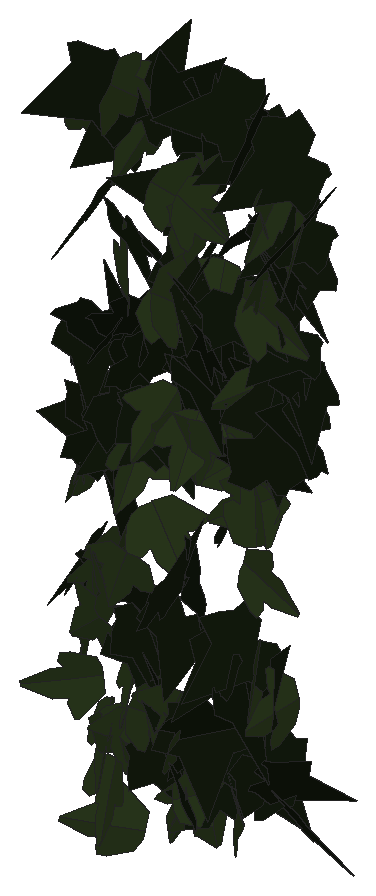
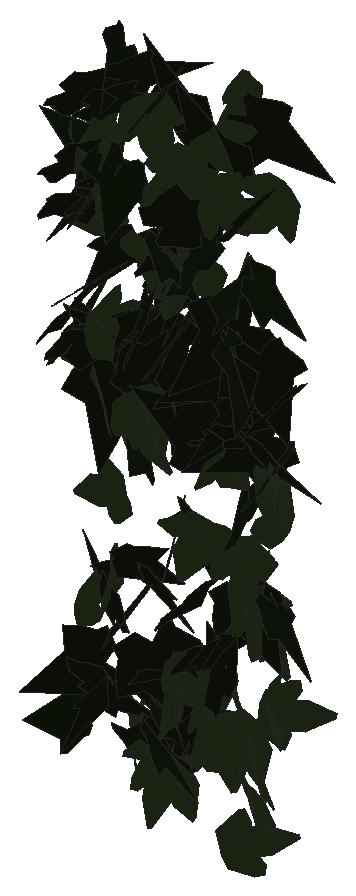
# SketchUp Ruby script. Lengths in inches.
U = 1.inch
M = Sketchup.active_model
def pt(a) = Geom::Point3d.new(a.map { |v| v * U })
def face(e, loops, mat)
  f = e.add_face(loops[0].map { |a| pt(a) })
  loops[1..].each { |l| e.add_face(l.map { |a| pt(a) }).erase! }
  f.material = f.back_material = mat if mat
  f
end
# faces: each face lists its corners as indices into pts; further lists are holes
def faces(e, pts, list, mat = nil) = list.each { |f| face(e, (f[0].is_a?(Array) ? f : [f]).map { |l| l.map { |i| pts[i] } }, mat) }
# xy, xz, yz: faces in a plane at the given z, y or x. An outline is a flat list of corners, or four numbers for a rectangle; further outlines are holes
def ring(l) = l.size == 4 ? [[l[0], l[1]], [l[2], l[1]], [l[2], l[3]], [l[0], l[3]]] : l.each_slice(2).to_a
def flat(e, list, mat, &to3) = list.each { |f| face(e, (f[0].is_a?(Array) ? f : [f]).map { |l| ring(l).map { |u, v| to3.(u, v) } }, mat) }
def xy(e, z, list, mat = nil) = flat(e, list, mat) { |x, y| [x, y, z] }
def xz(e, y, list, mat = nil) = flat(e, list, mat) { |x, z| [x, y, z] }
def yz(e, x, list, mat = nil) = flat(e, list, mat) { |y, z| [x, y, z] }
def lines(e, pts, list) = list.each { |a, b| e.add_line(pt(pts[a]), pt(pts[b])) }
# prism: a flat outline (further loops are holes) pulled along v
def prism(e, loops, v, mat = nil)
  f = face(e, loops, mat); d = Geom::Vector3d.new(v.map { |x| x * U })
  f.pushpull(f.normal.samedirection?(d) ? d.length : -d.length)
end
def box(e, o, s, mat = nil) = prism(e, [[o, [o[0] + s[0], o[1], o[2]], [o[0] + s[0], o[1] + s[1], o[2]], [o[0], o[1] + s[1], o[2]]]], [0, 0, s[2]], mat)
def at(x, y, z, deg = 0) = Geom::Transformation.translation(pt([x, y, z])) * Geom::Transformation.rotation(ORIGIN, Z_AXIS, deg.degrees)
def axes(o, x, y, z) = Geom::Transformation.new([*x, 0, *y, 0, *z, 0, *pt(o).to_a, 1])
def part(name) = M.definitions.add(name)
# library, detail: a bought-in or finely detailed component or shape, given as its bounding box
def library(name, o, s) = part(name).tap { |d| box(d.entities, o, s) }
def detail(e, o, s) = box(e.add_group.entities, o, s)
def put(e, d, t, mat = nil) = e.add_instance(d, t).tap { |i| i.material = mat if mat }
def group(e, t, mat = nil) = e.add_group.tap { |g| g.transformation = t; g.material = mat if mat }.entities
root = M.entities
M.materials.add("efeu1").color = [18, 25, 13]
M.materials.add("efeu2").color = [43, 57, 29]
c1 = part("ivyleaf_9")
p = [[1.54,2.16,1.25],[1.36,2.04,1.19],[-0.21,0.99,0.68],[-0.71,1.11,0.82],[-0.85,0.86,0.67],[-0.8,0.17,0.21],
  [-0.9,-0.01,0.1],[-0.67,-0.16,-0.02],[-0.08,-0.08,-0.05],[-0.03,-0.6,-0.4],[0.65,-0.88,-0.66],[0.83,-0.6,-0.49],
  [1.29,-0.42,-0.43],[1.8125,-0.07,-0.26],[1.21,0.44,0.15]]
faces(c1.entities,p,[[0,1,2,3,4,5,6,7,8,9,10,11,12,13,14]],"efeu1")
c2 = part("ivyleaf_10")
p = [[0,0.5,-0.03],[-0.0625,2.02,-0.43],[-0.19,2.01,-0.46],[-0.54,1.05,-0.29],[-0.52,0.625,-0.18],[-0.83,0.76,-0.28],
  [-1.16,0.64,-0.33],[-1.15,0.33,-0.24],[-0.77,-0.39,0.02],[-0.3,-0.51,0.16],[0.04,-0.48,0.23],[-0.02,2.01,-0.4375],
  [-0.06,2.01,-0.43],[0.04,-0.49,0.23],[0.67,-0.49,0.14],[1.38,0.36,-0.2],[1.375,0.51,-0.24],[0.81,0.65,-0.19],
  [0.62,0.59,-0.15],[0.6,1.09,-0.28],[0.5,1.23,-0.31]]
faces(c2.entities,p,[[0,1,2,3,4,5,6,7,8,9,10],[11,12,0,13,14,15,16,17,18,19,20]],"efeu2")
put(root,c1,axes([540.07,132.12,190.23],[-0.77853,0.07649,-0.13455],[0.13481,-0.0038,-0.78222],[-0.07602,-0.79006,-0.00927]))
put(root,c1,axes([536.34,132.2,205.77],[-0.01479,-0.04533,-0.99131],[-0.70127,-0.70098,0.04252],[-0.70211,0.7011,-0.02159]))
put(root,c2,axes([541.32,131.96,195.22],[0.4673,0.11071,-0.69672],[-0.70545,0.07863,-0.46066],[0.00448,0.83523,0.13572]))
put(root,c1,axes([538.57,131.37,191.45],[-0.5534,0.68611,-0.1935],[-0.12157,0.15055,0.88148],[0.70243,0.5666,0.00011]))
put(root,c2,axes([541.42,131.6,194.71],[-0.0205,0.8887,-0.32651],[-0.00715,0.32643,0.88893],[0.94675,0.02171,-0.00036]))
put(root,c2,axes([536.9,132,191.92],[-0.72646,-0.1609,0.31255],[-0.29232,-0.12205,-0.74228],[0.19526,-0.78137,0.05159]))
put(root,c2,axes([541.12,132,200.8],[0.26644,-0.01284,0.95425],[0.94592,0.13486,-0.2623],[-0.12648,0.98153,0.04852]))
put(root,c2,axes([539.0625,132.14,196.57],[0.51752,0.59596,-0.26554],[-0.17048,-0.20364,-0.78929],[-0.62977,0.54486,-0.00455]))
put(root,c2,axes([538,132.46,196.8],[-0.31807,-0.61315,0.55252],[-0.04869,-0.57716,-0.66852],[0.82393,-0.27081,0.17379]))
put(root,c1,axes([539.3125,131.78,199.68],[0.65022,0.02162,-0.51347],[-0.5119,-0.04616,-0.65018],[-0.04556,0.82723,-0.02286]))
put(root,c1,axes([541.74,131.8,196.24],[-0.50867,-0.16923,0.60195],[0.59928,0.08952,0.53158],[-0.17846,0.78299,0.06932]))
put(root,c2,axes([539.14,131.94,196.61],[-0.86929,-0.17236,0.04788],[-0.04691,-0.00958,-0.88622],[0.17262,-0.87056,0.00027]))
put(root,c2,axes([541.65,132.66,189.07],[-0.17144,0.03539,0.8404],[0.22296,-0.82509,0.08023],[0.81106,0.23429,0.15558]))
put(root,c2,axes([537.01,131.5625,206.11],[0.00032,-0.58195,-0.70668],[0.2085,0.68816,-0.5666],[0.8914,-0.16075,0.13278]))
put(root,c2,axes([535.1,132.65,194.67],[-0.18261,0.1429,-0.82601],[0.22635,-0.80557,-0.18941],[-0.80714,-0.25825,0.13376]))
put(root,c1,axes([540.64,132.61,190.62],[-0.64258,-0.4605,0.26493],[-0.20561,-0.16781,-0.79039],[0.48987,-0.67449,0.01577]))
put(root,c2,axes([538.71,131.42,200.5625],[-0.16647,0.55936,0.8349],[-0.21855,0.80588,-0.58349],[-0.98091,-0.27448,-0.01169]))
put(root,c1,axes([540.25,132.39,189.18],[0.4111,-0.79665,0.03566],[0.02292,-0.0283,-0.89643],[0.79712,0.41167,0.00739]))
put(root,c1,axes([537.89,132.625,200.7],[0.17256,-0.63262,0.66271],[0.46155,-0.52251,-0.61897],[0.79143,0.44265,0.21648]))
put(root,c2,axes([536.12,132.25,190.52],[-0.46099,0.62911,0.2138],[0.12797,-0.17128,0.77993],[0.652,0.47842,-0.00192]))
put(root,c2,axes([536.03,132.02,189.94],[-0.48907,0.03641,0.64444],[-0.64379,0.03067,-0.49031],[-0.04645,-0.80842,0.01042]))
put(root,c2,axes([535.25,132.49,187.72],[0.05497,0.09973,-0.81363],[-0.72569,-0.37331,-0.09478],[-0.38121,0.72503,0.06312]))
put(root,c2,axes([537.02,132.43,195.01],[0.30457,0.63822,-0.40303],[-0.14524,-0.37693,-0.70665],[-0.74072,0.33634,-0.02716]))
put(root,c2,axes([541.41,132.21,201.97],[0.22118,-0.82992,-0.15972],[-0.02563,0.15843,-0.85875],[0.84476,0.2221,0.01576]))
put(root,c2,axes([541.39,132.68,203.86],[0.06859,0.59315,-0.69627],[-0.12261,-0.68596,-0.59644],[-0.90641,0.13767,0.02799]))
put(root,c2,axes([539,132.33,202.625],[-0.63997,-0.4633,0.24883],[-0.17815,-0.17777,-0.78917],[0.4948,-0.66323,0.0377]))
put(root,c1,axes([536.07,131.6875,195.63],[0.13792,0.13266,-0.84326],[0.16931,0.83297,0.15873],[0.83667,-0.19043,0.10688]))
put(root,c2,axes([538.26,131.8125,200.13],[0.35067,0.4968,0.56306],[0.19816,0.53818,-0.59826],[-0.72428,0.38778,0.10893]))
put(root,c1,axes([540.29,132.75,205.88],[-0.49246,-0.10914,0.68792],[-0.58927,-0.38391,-0.48275],[0.37137,-0.7539,0.14624]))
put(root,c1,axes([541.21,131.58,205.94],[-0.25357,0.2213,-0.84943],[-0.65638,0.53924,0.33642],[0.5828,0.7036,0.00933]))
put(root,c1,axes([538.68,132.37,185.375],[0.27035,-0.6387,0.36456],[-0.05983,0.36803,0.68914],[-0.73299,-0.26562,0.07821]))
put(root,c1,axes([541.7,131.79,202.29],[-0.07841,0.95808,0.01706],[-0.00503,-0.01753,0.96126],[0.95822,0.0783,0.00644]))
put(root,c2,axes([540.83,132.68,190.06],[-0.13952,0.47632,-0.68271],[0.1207,-0.67334,-0.49445],[-0.82366,-0.17936,0.04319]))
put(root,c1,axes([538.72,132.625,198.1],[0.36217,-0.79476,0.17443],[0.09397,-0.14879,-0.87308],[0.80823,0.37343,0.02335]))
put(root,c1,axes([538.77,132.69,201],[-0.18331,-0.80207,-0.03123],[0.00884,0.03001,-0.82274],[0.80263,-0.18351,0.00193]))
put(root,c1,axes([538.13,132.875,190.27],[-0.11478,-0.79669,0.27399],[0.02385,-0.27949,-0.80267],[0.84215,-0.10067,0.06008]))
put(root,c1,axes([537.15,132.82,195.75],[-0.6646,-0.3726,0.30722],[-0.23086,-0.21391,-0.75885],[0.42417,-0.70023,0.06834]))
put(root,c2,axes([538.25,132.45,188.13],[-0.55106,-0.46259,0.30455],[-0.23513,-0.19358,-0.71948],[0.50146,-0.59912,-0.00268]))
put(root,c2,axes([539.14,131.82,203.28],[-0.00881,0.67359,0.56678],[-0.01403,0.56663,-0.67363],[-0.88021,-0.01577,0.00506]))
put(root,c1,axes([538.58,132.93,191.48],[0.00451,-0.20055,0.79906],[0.0062,-0.79904,-0.20058],[0.82382,0.00711,-0.00287]))
put(root,c1,axes([539.5,132.41,188.26],[-0.01946,0.71355,-0.61813],[-0.06258,-0.61788,-0.71129],[-0.94198,0.0263,0.06002]))
put(root,c1,axes([539.05,132.625,187.7],[-0.20607,-0.81278,-0.24845],[0.05444,0.2425,-0.83847],[0.84816,-0.21304,-0.00654]))
put(root,c2,axes([538.32,131.8125,203.45],[0.13862,0.49802,0.65345],[-0.0052,0.6632,-0.50435],[-0.82158,0.07983,0.11344]))
put(root,c2,axes([539.87,132.77,185.29],[-0.27744,0.16552,0.85045],[0.73133,-0.43407,0.32306],[0.46456,0.78218,-0.00068]))
put(root,c2,axes([542.08,132.58,203.11],[0.58485,-0.70705,0.10192],[0.06833,-0.07575,-0.91757],[0.71108,0.58881,0.00435]))
put(root,c1,axes([541.14,132.93,202.21],[0.13954,-0.67261,0.56712],[0.32375,-0.49466,-0.66633],[0.81805,0.3105,0.16697]))
put(root,c1,axes([540.89,132.45,188.85],[-0.30926,0.43987,0.64221],[0.30279,-0.56864,0.53529],[0.71711,0.4298,0.05094]))
put(root,c1,axes([542.1,133,197.05],[0.45563,-0.7397,-0.20503],[0.11152,-0.17211,0.86875],[-0.75944,-0.46905,0.00456]))
put(root,c1,axes([541.85,133.1,205.07],[-0.63778,-0.50586,0.51395],[-0.36402,-0.36645,-0.8124],[0.62252,-0.73254,0.05149]))
put(root,c2,axes([535.26,132.29,193.65],[0.28992,-0.90055,0.27936],[-0.08657,0.26561,0.94607],[-0.9389,-0.30256,-0.00097]))
put(root,c1,axes([535.84,133.03,193.72],[0.16767,-0.62273,0.60556],[0.15712,-0.58482,-0.6449],[0.85429,0.22978,-0.00024]))
put(root,c1,axes([536.51,131.99,196.7],[0.21578,-0.20512,-0.76242],[-0.19529,0.75196,-0.25757],[0.765,0.24982,0.1493]))
put(root,c2,axes([535.85,132.66,185],[0.79693,-0.40304,0.19952],[0.17322,-0.09954,-0.89299],[0.41502,0.81547,-0.0104]))
put(root,c1,axes([539.44,132.45,198.35],[0.32395,0.5127,-0.62044],[-0.33352,-0.52318,-0.60647],[-0.73252,0.46495,0.00174]))
put(root,c2,axes([540.7,133.2,198.08],[-0.04711,0.03685,0.93794],[0.02759,-0.93866,0.03827],[0.93825,0.02946,0.04597]))
put(root,c1,axes([540.27,132.32,200.73],[0.07173,-0.53209,-0.65439],[0.08721,0.65791,-0.52539],[0.83889,-0.0229,0.11057]))
put(root,c1,axes([535.98,132.375,195.56],[-0.56947,0.40005,0.5151],[-0.45389,0.24796,-0.69438],[-0.46835,-0.72673,0.04663]))
put(root,c2,axes([540.7,132.51,192.66],[0.23601,-0.00578,0.78886],[0.78092,0.11838,-0.23277],[-0.11178,0.81485,0.03941]))
put(root,c2,axes([536.92,131.95,200.07],[-0.16704,0.36092,-0.85968],[-0.35195,0.78434,0.39768],[0.86339,0.38956,-0.00421]))
put(root,c2,axes([536.46,132.81,188.32],[0.53537,-0.46618,0.2947],[0.21534,-0.20142,-0.70983],[0.50774,0.57697,-0.00969]))
put(root,c1,axes([538.01,132.59,205.03],[-0.34339,0.36354,0.87223],[0.59923,-0.63381,0.50008],[0.73067,0.69064,-0.0002]))
put(root,c1,axes([535.74,132.48,198.61],[0.26462,0.55929,-0.58872],[-0.36306,-0.47236,-0.61194],[-0.72634,0.43987,0.0914]))
put(root,c2,axes([536.19,132.99,183.4375],[0.11513,0.14111,0.83023],[-0.51154,-0.65393,0.18208],[0.66897,-0.52432,-0.00365]))
put(root,c1,axes([540.95,133.21,205.02],[-0.56399,-0.36253,0.53342],[-0.36073,-0.41009,-0.66011],[0.53464,-0.65912,0.11732]))
put(root,c2,axes([541.17,132.5,194.89],[0.74121,-0.48035,0.11053],[-0.08554,0.07122,0.88315],[-0.48543,-0.74601,0.01315]))
put(root,c2,axes([537.42,132,187.72],[0.02966,0.43063,0.7255],[-0.1629,0.71521,-0.41787],[-0.8278,-0.12531,0.10822]))
put(root,c1,axes([540.9,132.3125,196.29],[0.72805,0.41398,-0.46611],[-0.4127,-0.21707,-0.83741],[-0.46725,0.83678,0.01336]))
put(root,c1,axes([539.08,133.29,205.47],[-0.10003,-0.61858,0.60768],[0.12877,-0.61552,-0.60536],[0.85751,0.02027,0.16179]))
put(root,c2,axes([536.06,132.58,186.625],[-0.66174,0.05436,-0.61325],[0.60841,-0.08004,-0.66361],[-0.09422,-0.89865,0.02201]))
put(root,c1,axes([537.64,132.52,186.59],[0.01246,-0.54744,-0.54993],[-0.02467,0.54944,-0.54751],[0.77556,0.02628,-0.00858]))
put(root,c1,axes([536.6,132.08,199.09],[0.76963,0.48589,0.25316],[0.20015,0.15701,-0.90984],[-0.51002,0.79484,0.02497]))
put(root,c1,axes([539.01,132.72,201.24],[-0.57239,0.52634,-0.30745],[0.2037,-0.23235,-0.77699],[-0.57452,-0.60677,0.03083]))
put(root,c1,axes([534.9,133.07,197.51],[0.06016,-0.78991,0.12088],[0.01914,-0.11977,-0.79214],[0.79888,0.06236,0.00987]))
put(root,c2,axes([539.4,132.76,200.86],[0.84043,0.01766,0.03566],[0.03574,-0.00354,-0.84061],[-0.01749,0.84118,-0.00428]))
put(root,c1,axes([541.48,132.24,186.97],[0.61151,0.23935,0.46236],[0.44094,0.14114,-0.65624],[-0.27683,0.75352,-0.02394]))
put(root,c2,axes([535.91,132.98,191.81],[0.0291,-0.80641,0.29743],[0.02433,-0.2967,-0.80683],[0.85916,0.03571,0.01277]))
put(root,c1,axes([537.58,132.69,196.58],[-0.30746,-0.55281,-0.6408],[0.31622,0.55735,-0.63254],[0.785,-0.44103,0.00383]))
put(root,c1,axes([539.27,133.08,196.89],[0.21068,0.17972,0.82727],[-0.7261,-0.39996,0.27181],[0.43527,-0.75419,0.05299]))
put(root,c1,axes([536.22,132.64,191.14],[0.23119,0.32532,-0.72399],[-0.5789,-0.44678,-0.38561],[-0.54301,0.61481,0.10287]))
put(root,c1,axes([534.94,133.05,195.42],[0.29532,-0.75516,0.18422],[0.10204,-0.1577,-0.81003],[0.77058,0.31029,0.03666]))
put(root,c1,axes([540.28,132.09,194.3],[-0.01983,0.42959,0.71938],[-0.11746,0.71105,-0.42785],[-0.82961,-0.11094,0.04338]))
put(root,c2,axes([538.7,132.27,187.625],[-0.01977,-0.65704,-0.66897],[-0.01226,0.66924,-0.65694],[0.93758,-0.0051,-0.0227]))
put(root,c1,axes([536.5,133.21,188.26],[0.04133,-0.22693,0.8247],[0.33553,-0.75519,-0.22461],[0.7868,0.33397,0.05246]))
put(root,c2,axes([536.67,132.82,186.82],[-0.585,-0.63572,0.1325],[-0.08238,-0.10424,-0.86387],[0.64413,-0.59069,0.00985]))
put(root,c2,axes([541,132.46,203.94],[-0.4364,0.67345,0.28048],[-0.196,0.20659,-0.80097],[-0.7027,-0.47585,0.04922]))
put(root,c1,axes([541.17,133.125,197.82],[-0.26019,-0.93373,-0.2218],[0.04606,0.2174,-0.9692],[0.9586,-0.26388,-0.01363]))
put(root,c2,axes([535.66,132.87,191.12],[-0.2313,-0.76503,0.07082],[-0.02235,-0.06722,-0.79923],[0.76798,-0.23236,-0.00193]))
put(root,c1,axes([536.76,133,189.67],[0.17286,-0.81229,-0.14974],[-0.02299,0.14819,-0.83044],[0.82565,0.17419,0.00823]))
put(root,c1,axes([535.11,132.75,191.2],[-0.52681,0.57154,-0.16378],[0.11019,-0.12118,-0.7773],[-0.58425,-0.53821,0.00109]))
put(root,c1,axes([541.4,132.77,202.04],[0.57782,-0.57472,-0.19355],[-0.11088,0.16271,-0.81417],[0.59621,0.58725,0.03616]))
put(root,c1,axes([541.61,132.76,197.71],[-0.5251,0.32717,0.51336],[-0.50615,0.14201,-0.60823],[-0.33821,-0.72048,0.11323]))
put(root,c1,axes([541.88,133.43,203.03],[-0.50996,-0.5231,0.43537],[-0.25453,-0.35796,-0.72823],[0.63119,-0.56698,0.05809]))
put(root,c2,axes([539.38,132.85,205.22],[-0.67646,-0.40888,0.27236],[-0.2477,-0.11641,-0.78997],[0.42427,-0.71989,-0.02695]))
put(root,c1,axes([536.9375,133.16,189.47],[-0.12866,-0.90428,-0.14311],[0.0323,0.13995,-0.91331],[0.91496,-0.1321,0.01212]))
put(root,c2,axes([535.33,133.17,186.33],[0.65508,-0.50287,0.45753],[0.36239,-0.27931,-0.82584],[0.57523,0.74863,-0.00077]))
put(root,c2,axes([537.9,133.28,186.64],[0.44852,-0.38571,0.7117],[0.57399,-0.4222,-0.59054],[0.57081,0.72762,0.0346]))
put(root,c1,axes([541.63,133.3,202.06],[-0.27654,-0.80923,-0.02822],[0.00887,0.02679,-0.85518],[0.80967,-0.27669,-0.00028]))
put(root,c1,axes([537.09,132.67,195.51],[0.0252,0.01828,0.98426],[0.97182,-0.15753,-0.02196],[0.15704,0.9719,-0.02207]))
put(root,c2,axes([538.73,132.34,185.46],[-0.00892,-0.05803,0.78167],[0.2076,0.75363,0.05832],[-0.75583,0.20768,0.0068]))
put(root,c1,axes([536.9,132.27,197.84],[0.06565,0.26502,-0.77192],[-0.07119,0.77332,0.25945],[0.81304,0.04631,0.08504]))
put(root,c1,axes([541.48,133,185.75],[0.6421,-0.41493,0.35933],[0.31753,-0.17027,-0.76404],[0.44772,0.71583,0.02654]))
put(root,c1,axes([539.04,133.47,198.9],[0.04557,-0.79307,0.36204],[0.15686,-0.34916,-0.7846],[0.85757,0.10601,0.12427]))
put(root,c1,axes([540.59,132.4,202.89],[0.08324,0.80238,0.26686],[0.00543,0.26764,-0.80641],[-0.84557,0.08071,0.0211]))
put(root,c1,axes([536.23,132.39,198.34],[-0.03485,0.7785,0.36985],[0.00147,0.3702,-0.77911],[-0.86189,-0.03085,-0.01628]))
put(root,c2,axes([538.23,133.27,185.23],[-0.12978,-0.76739,0.29801],[-0.05593,-0.29277,-0.77827],[0.82132,-0.1412,-0.00591]))
put(root,c1,axes([539.17,133.6875,198.5],[0.04027,-0.43997,0.81692],[0.09744,-0.81116,-0.44167],[0.92273,0.10486,0.01099]))
put(root,c1,axes([541.32,133.02,186.72],[-0.61799,0.23459,0.61311],[-0.57901,0.20199,-0.66091],[-0.30932,-0.84677,0.01221]))
put(root,c2,axes([536.66,133.26,205.46],[0.51747,0.47535,-0.46251],[-0.36501,-0.28569,-0.70199],[-0.55375,0.63251,0.03052]))
put(root,c1,axes([541.12,133.76,199.39],[-0.42495,-0.61016,0.47435],[0.02288,-0.55102,-0.68828],[0.77251,-0.31932,0.28132]))
put(root,c2,axes([534.74,132.99,204.2],[-0.66957,0.04161,-0.52033],[0.51825,-0.04814,-0.67075],[-0.06237,-0.84661,0.01257]))
put(root,c1,axes([535.78,133.41,200.88],[0.40631,-0.63201,0.30507],[0.16262,-0.25812,-0.75135],[0.68269,0.43764,-0.00258]))
put(root,c2,axes([534.51,133.49,188.5],[0.38862,-0.53363,0.52554],[0.36383,-0.38302,-0.65795],[0.65466,0.52964,0.05369]))
put(root,c1,axes([541.63,133.53,198.53],[0.13055,-0.8422,0.12492],[0.01773,-0.12366,-0.85226],[0.85123,0.13175,-0.00141]))
put(root,c1,axes([536.79,132.89,204.625],[-0.6704,0.37527,0.63127],[0.55127,-0.30757,0.76828],[0.48521,0.86795,-0.00068]))
put(root,c2,axes([536.39,133.58,203.87],[-0.11646,-0.64906,0.53325],[0.00342,-0.53871,-0.65496],[0.84001,-0.0878,0.07659]))
put(root,c2,axes([539.63,133.13,195.4],[0.54843,-0.15889,-0.54624],[-0.53247,0.1237,-0.57059],[0.20024,0.7641,-0.02121]))
put(root,c1,axes([536.49,132.74,197.6],[0.05788,-0.03016,0.91369],[-0.41275,0.81603,0.05309],[-0.8157,-0.41505,0.03798]))
put(root,c2,axes([537.22,132.96,192.86],[0.67596,0.47955,0.41645],[0.32158,0.26604,-0.82832],[-0.5477,0.74805,0.02762]))
put(root,c1,axes([538.16,133.57,202.375],[-0.23536,-0.07648,0.83036],[-0.7904,-0.2545,-0.24748],[0.26575,-0.8247,-0.00064]))
put(root,c2,axes([539.28,133.37,196.33],[-0.59975,-0.42821,0.35565],[-0.19569,-0.32723,-0.724],[0.52111,-0.61572,0.13744]))
put(root,c2,axes([538.77,133.06,185.04],[-0.29843,-0.73939,-0.21711],[0.09407,0.19612,-0.79723],[0.76484,-0.31263,0.01334]))
put(root,c1,axes([535.45,133.89,203.53],[-0.32091,-0.52157,0.60758],[-0.13917,-0.60827,-0.59566],[0.78856,-0.31961,0.14213]))
put(root,c1,axes([540.57,132.98,186.89],[0.2953,-0.55151,-0.5727],[-0.1533,0.55997,-0.6183],[0.78016,0.31879,0.09528]))
put(root,c1,axes([535.13,133.45,201.64],[-0.58105,0.36774,-0.43299],[0.26426,-0.37331,-0.67167],[-0.50287,-0.62108,0.14734]))
put(root,c1,axes([539.26,132.92,185.2],[-0.89378,0.11847,0.07707],[0.07427,-0.0261,0.90145],[0.12024,0.89672,0.01605]))
put(root,c1,axes([538.71,133.38,186.53],[-0.64347,0.50451,-0.44426],[0.35539,-0.26671,-0.81762],[-0.57061,-0.73504,-0.00825]))
